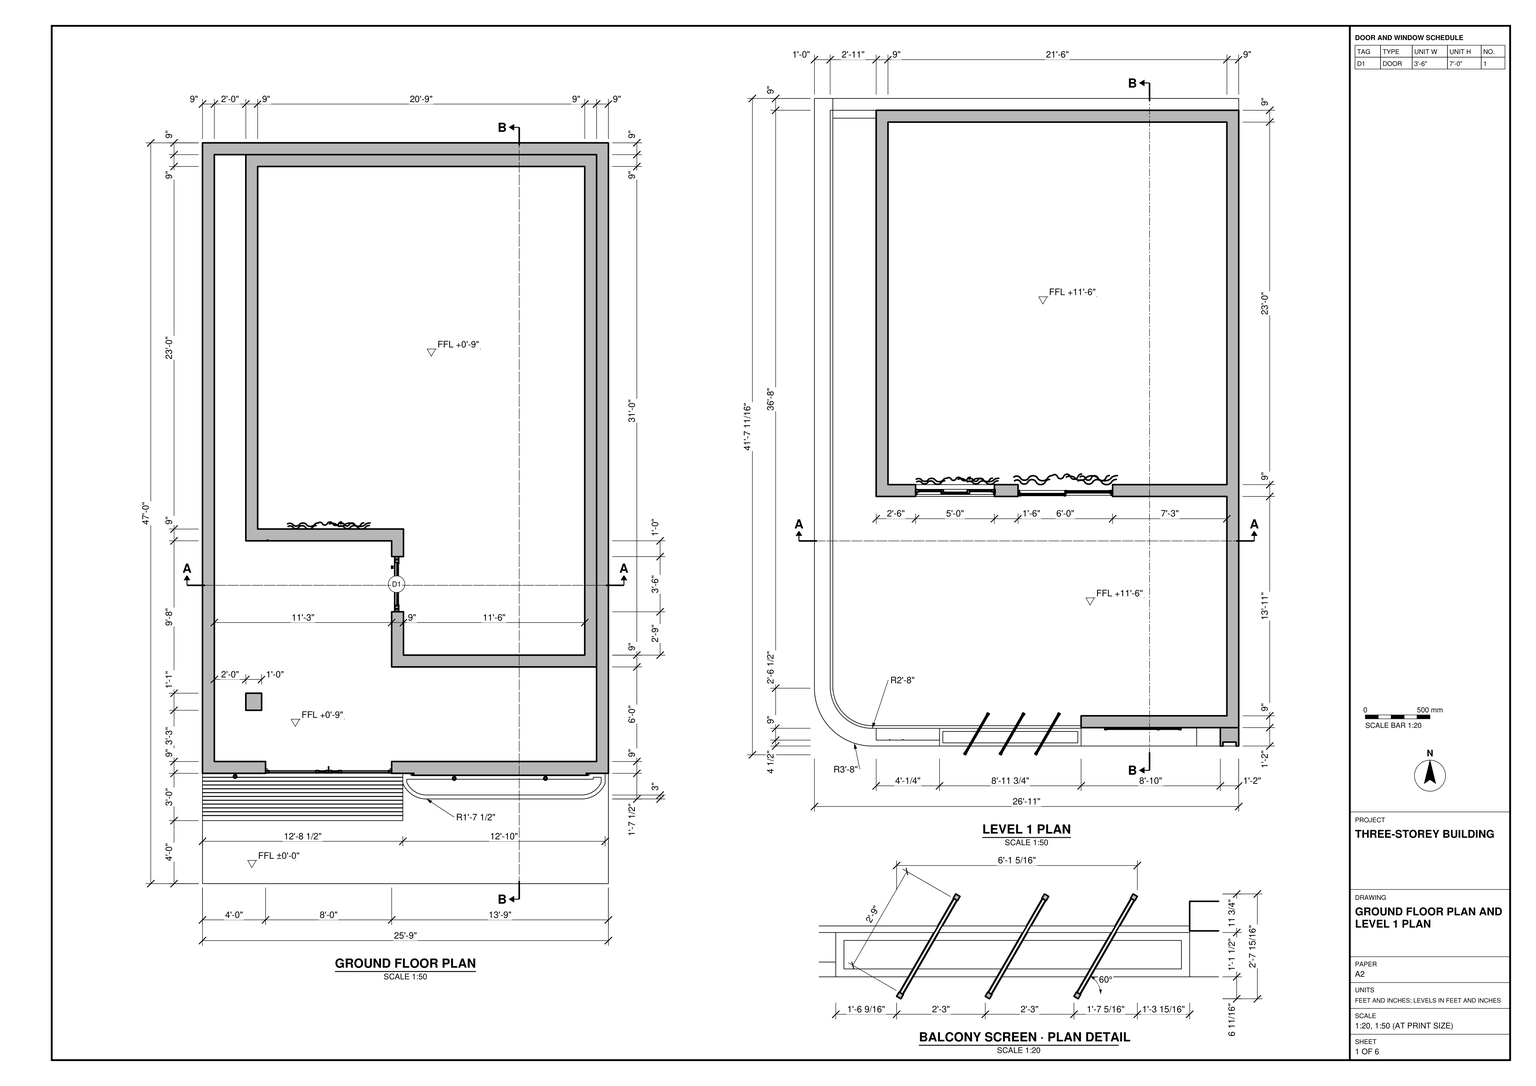
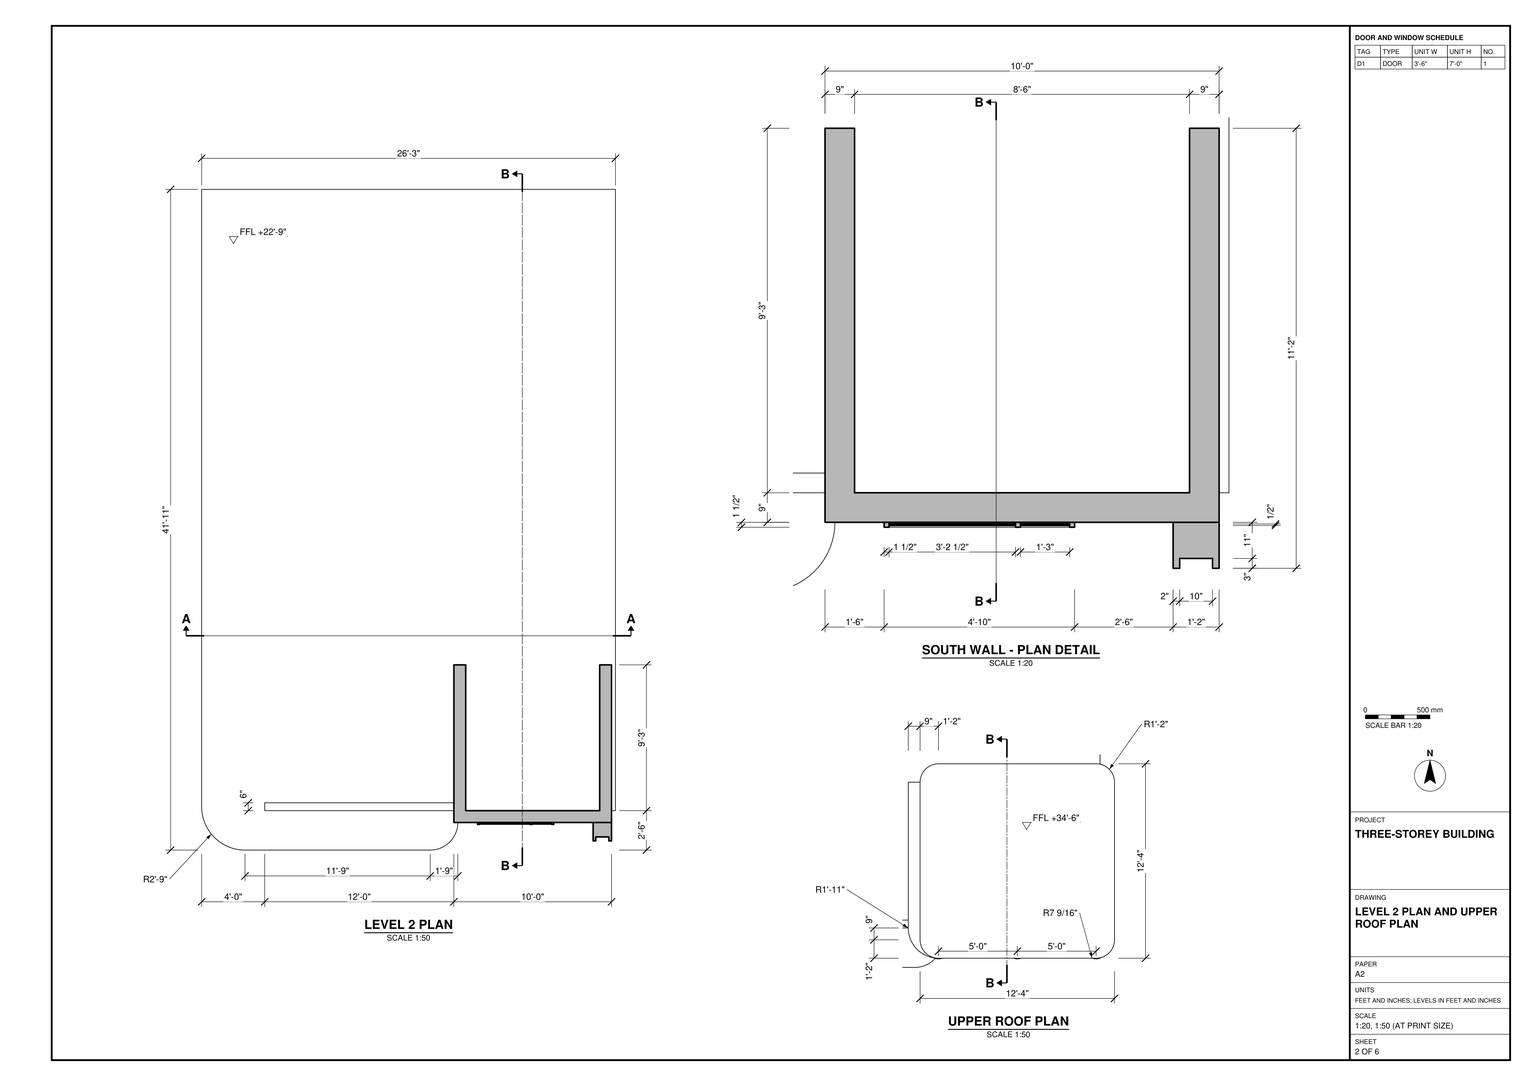
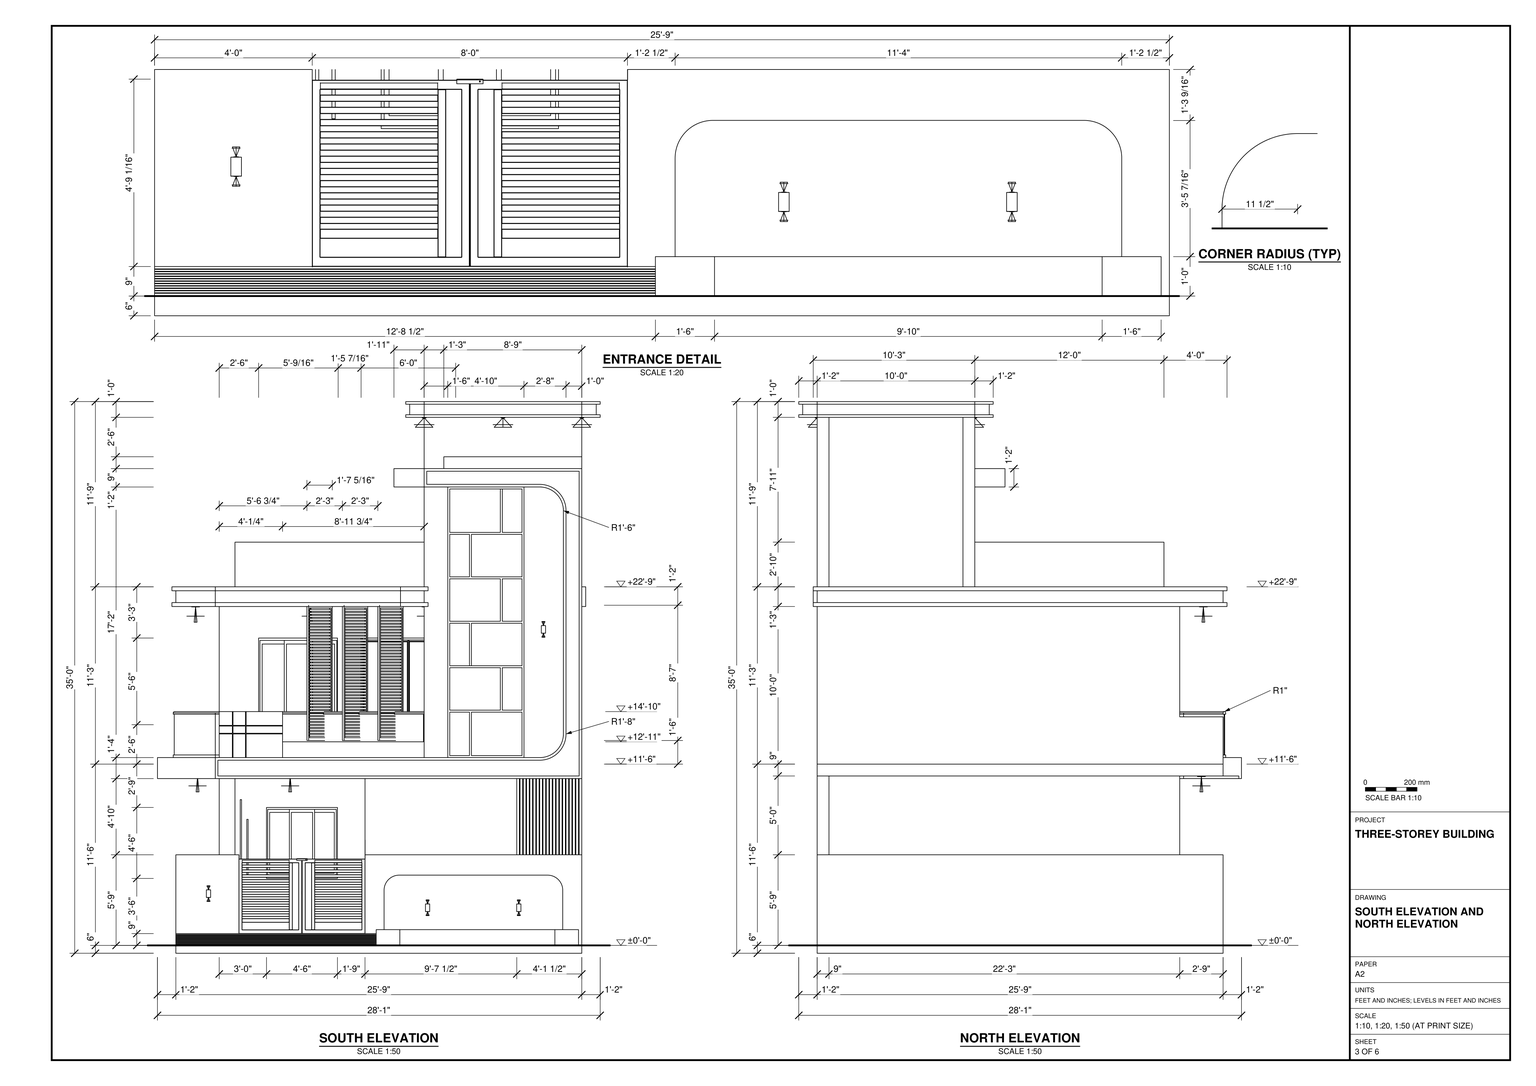
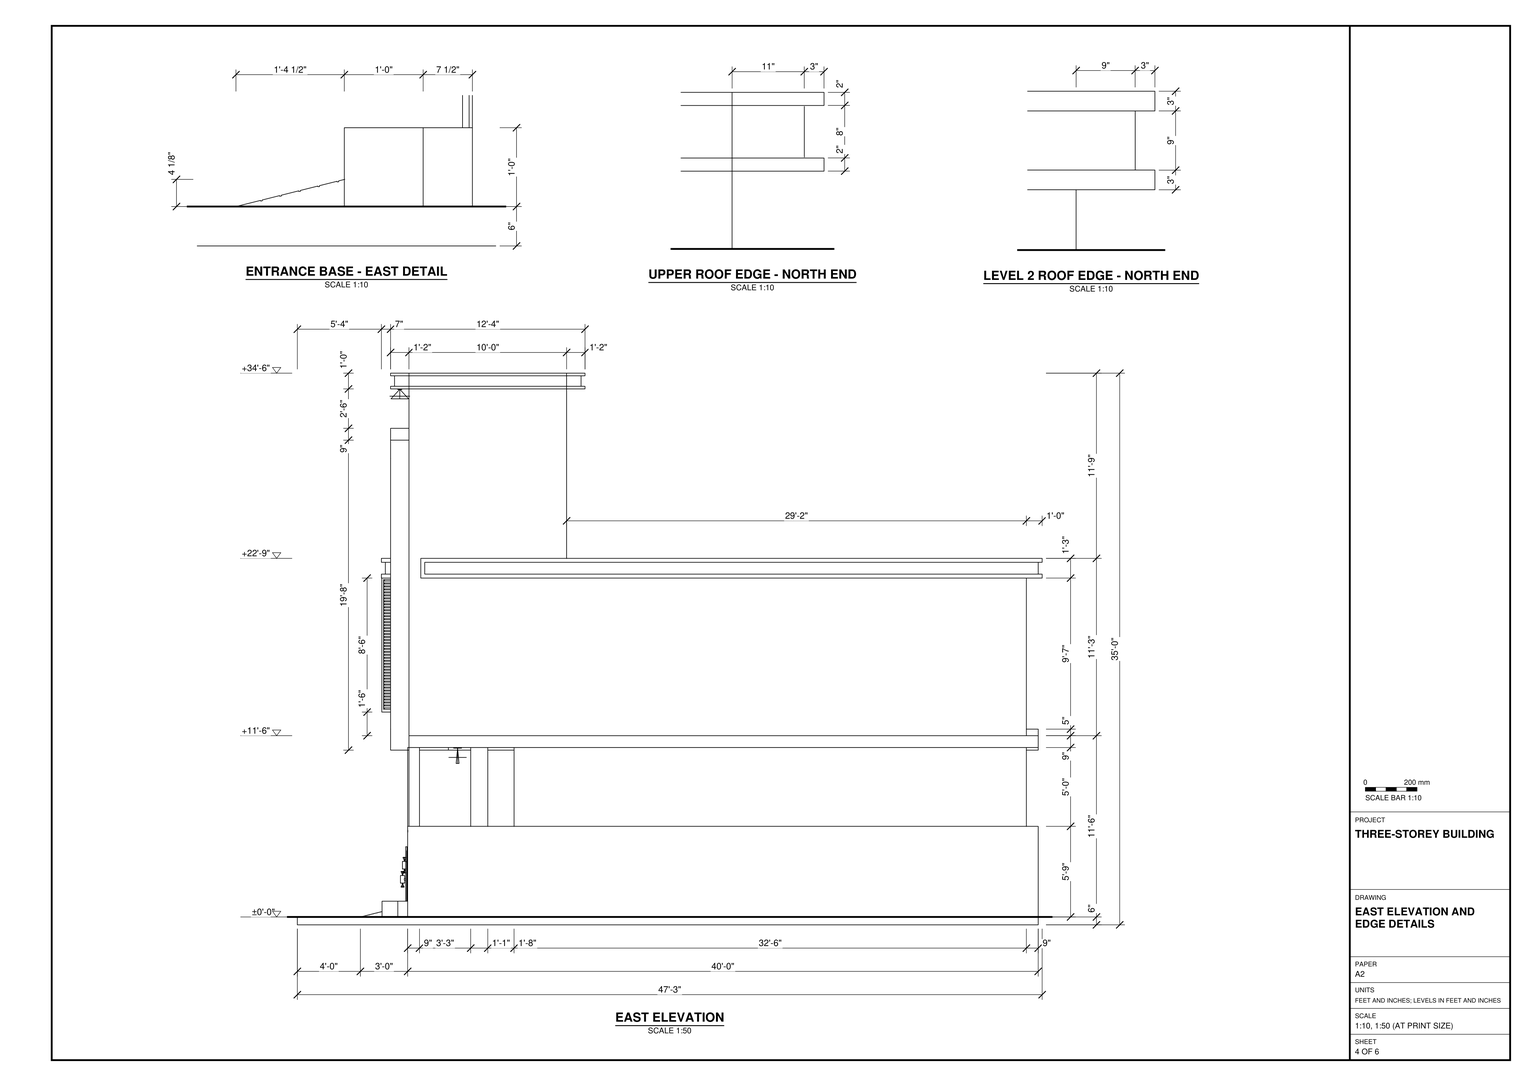
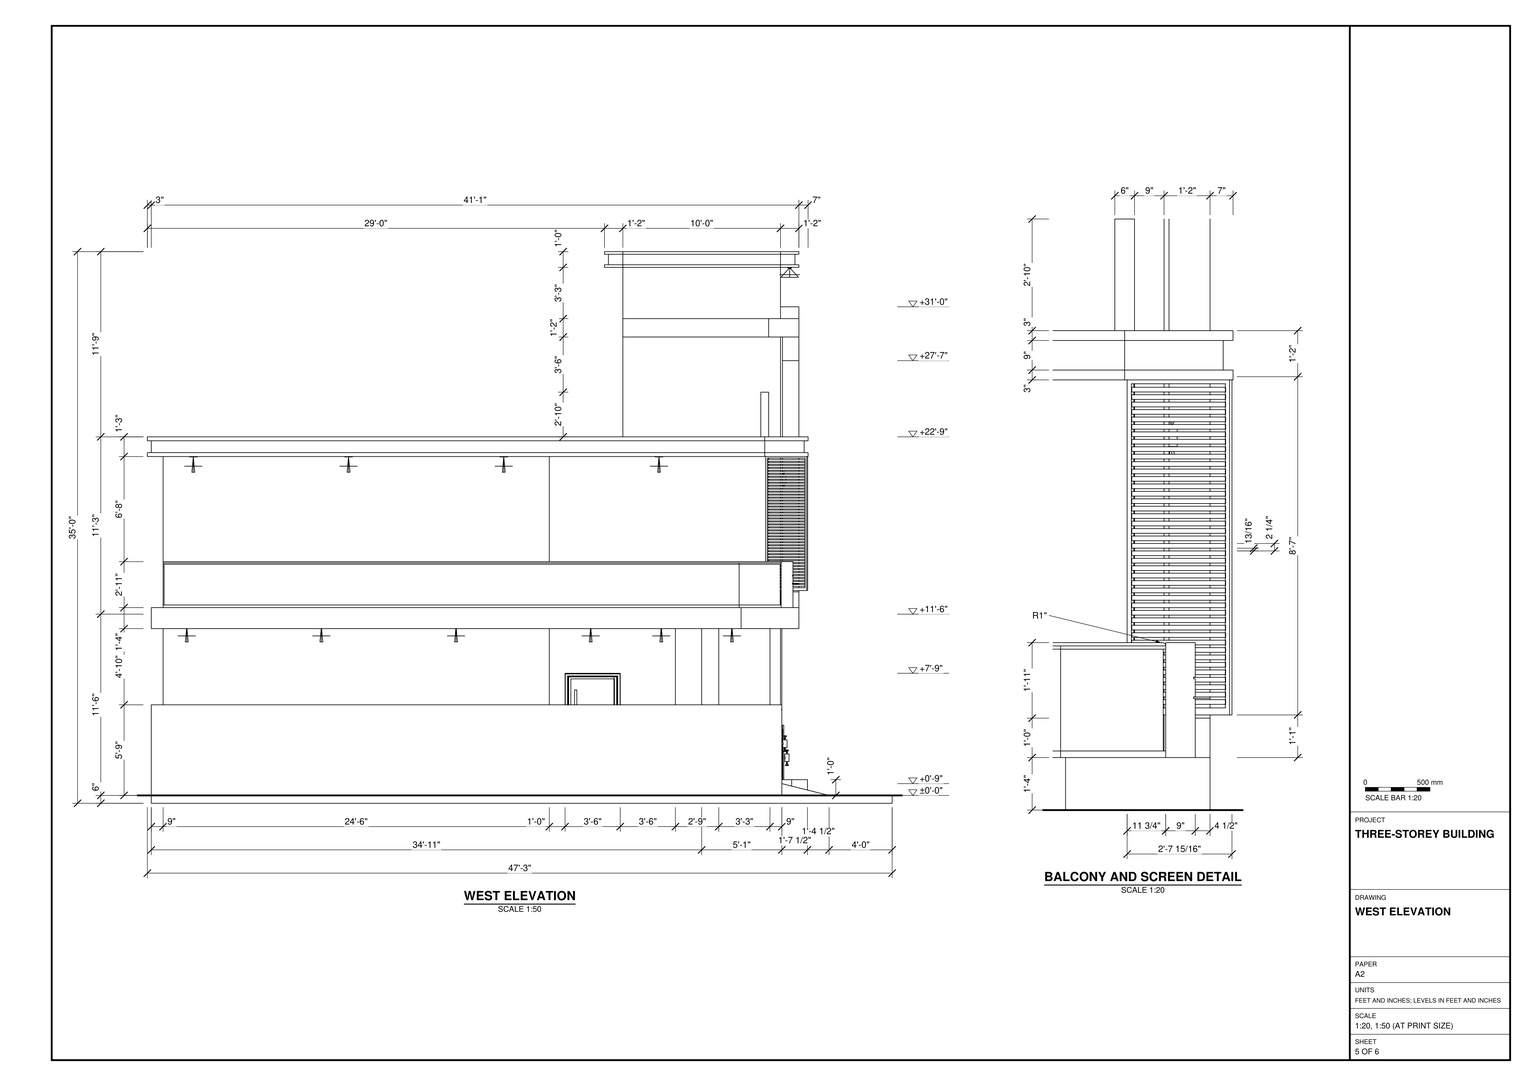
Build the three-storey building in SketchUp from task_files/diagram_01.pdf. Work in feet and inches. The overall model, including its projections, is 28'-1" wide, 47'-3" deep and 35'-0" high. Use ±0'-0" as the ground datum, with Level 1 at +11'-6" and Level 2 at +22'-9". Distinguish the raised ground-floor surface from the ground datum.

Follow the plan of each floor rather than repeating one footprint. Model the walls at their drawn thicknesses, including the 9" walls and the stepped ground-floor wall with a door in its return. On the south front, form the entrance steps, double slatted gate and adjoining low wall with its rounded-corner panel. Set the Level 1 enclosure back from the balcony. Include the window and door openings behind the balcony, the rounded slab corner, the railing and the angled slatted screens. Use the south elevation to place the tall panelled bay to the right of the screens and to shape its curved frame. At Level 2, model the broad roof deck and the smaller U-shaped wall at the front right, with its own overhanging roof cap.

Keep walls, slabs and roofs in separate groups or components. Group each furniture or joinery piece shown separately and use components for repeated parts. Decor and loose items, including light fixtures, may be any suitable library components. Save one SketchUp model as output_files/three_storey_building_with_a_screened_front_balcony.skp.

# SketchUp Ruby script. Lengths in inches.
U = 1.inch
M = Sketchup.active_model
def pt(a) = Geom::Point3d.new(a.map { |v| v * U })
def face(e, loops, mat)
  f = e.add_face(loops[0].map { |a| pt(a) })
  loops[1..].each { |l| e.add_face(l.map { |a| pt(a) }).erase! }
  f.material = f.back_material = mat if mat
  f
end
# faces: each face lists its corners as indices into pts; further lists are holes
def faces(e, pts, list, mat = nil) = list.each { |f| face(e, (f[0].is_a?(Array) ? f : [f]).map { |l| l.map { |i| pts[i] } }, mat) }
# xy, xz, yz: faces in a plane at the given z, y or x. An outline is a flat list of corners, or four numbers for a rectangle; further outlines are holes
def ring(l) = l.size == 4 ? [[l[0], l[1]], [l[2], l[1]], [l[2], l[3]], [l[0], l[3]]] : l.each_slice(2).to_a
def flat(e, list, mat, &to3) = list.each { |f| face(e, (f[0].is_a?(Array) ? f : [f]).map { |l| ring(l).map { |u, v| to3.(u, v) } }, mat) }
def xy(e, z, list, mat = nil) = flat(e, list, mat) { |x, y| [x, y, z] }
def xz(e, y, list, mat = nil) = flat(e, list, mat) { |x, z| [x, y, z] }
def yz(e, x, list, mat = nil) = flat(e, list, mat) { |y, z| [x, y, z] }
def lines(e, pts, list) = list.each { |a, b| e.add_line(pt(pts[a]), pt(pts[b])) }
# prism: a flat outline (further loops are holes) pulled along v
def prism(e, loops, v, mat = nil)
  f = face(e, loops, mat); d = Geom::Vector3d.new(v.map { |x| x * U })
  f.pushpull(f.normal.samedirection?(d) ? d.length : -d.length)
end
def box(e, o, s, mat = nil) = prism(e, [[o, [o[0] + s[0], o[1], o[2]], [o[0] + s[0], o[1] + s[1], o[2]], [o[0], o[1] + s[1], o[2]]]], [0, 0, s[2]], mat)
def at(x, y, z, deg = 0) = Geom::Transformation.translation(pt([x, y, z])) * Geom::Transformation.rotation(ORIGIN, Z_AXIS, deg.degrees)
def axes(o, x, y, z) = Geom::Transformation.new([*x, 0, *y, 0, *z, 0, *pt(o).to_a, 1])
def part(name) = M.definitions.add(name)
# library, detail: a bought-in or finely detailed component or shape, given as its bounding box
def library(name, o, s) = part(name).tap { |d| box(d.entities, o, s) }
def detail(e, o, s) = box(e.add_group.entities, o, s)
def put(e, d, t, mat = nil) = e.add_instance(d, t).tap { |i| i.material = mat if mat }
def group(e, t, mat = nil) = e.add_group.tap { |g| g.transformation = t; g.material = mat if mat }.entities
root = M.entities
M.materials.add("1496 AP 8293 CARBON COPY").color = [58, 58, 58]
M.materials.add("1755 AP K184 Brass Olive-N").color = [221, 212, 201]
M.materials.add("Antracyt").color = [44, 47, 50]
M.materials.add("Carpet_Frieze_Low").color = [170, 156, 146]
M.materials.add("Carpet_Loop_Low").color = [201, 172, 127]
M.materials.add("Wall Light").color = [248, 221, 148]
M.materials.add("[0135_DarkGray]").color = [81, 81, 81]
M.materials.add("[Basic Tile]").color = [188, 188, 188]
M.materials.add("[Carrera Marble]").color = [233, 230, 225]
M.materials.add("[Terrazzo Tile Light]").color = [178, 178, 178]
M.materials.add("[Translucent Glass Blue]").color = [169, 185, 212]
M.materials.add("[Translucent Glass Gray]").color = [128, 128, 128]
M.materials.add("[Wood Cherry Original]").color = [91, 49, 20]
M.materials.add("[Wood Cherry Original]1").color = [25, 25, 25]
c1 = library("2",[-4.69,-4.69,-13.16],[13.38,13.38,13.16])
c2 = library("WALL LIGHT 69",[4.19,4.05,-8.78],[4.61,5.7,17.13])
c3 = library("Group\#2",[0,-19.5,0],[309,499.5,129])
c4 = part("หน้าต่าง3บาน")
xy(c4.entities,42.78,[[77.6875,12.74,148.55,16.68]],"Antracyt")
xy(c4.entities,43.96,[[78.87,12.74,147.37,12.74,147.37,14.71,125.72,14.71,125.72,13.13,100.52,13.13,100.52,14.71,78.87,14.71],[100.52,13.13,102.88,14.71],[123.36,13.13,125.72,14.71],[102.49,14.71,123.75,14.71,123.75,16.28,147.37,16.28,147.37,16.68,78.87,16.68,78.87,16.28,102.49,16.28]],"Antracyt")
xy(c4.entities,45.93,[[102.49,13.13,123.75,13.92],[102.49,13.92,123.75,14.71],[80.84,14.71,100.52,15.49],[125.72,14.71,145.4,15.49],[80.84,15.49,100.52,16.28],
  [125.72,15.49,145.4,16.28]],"Antracyt")
xy(c4.entities,83.09,[[102.49,13.13,123.75,13.92],[102.49,13.92,123.75,14.71],[80.84,14.71,100.52,15.49],[125.72,14.71,145.4,15.49],[80.84,15.49,100.52,16.28],
  [125.72,15.49,145.4,16.28]],"Antracyt")
xy(c4.entities,84.91,[[78.87,12.74,78.87,14.71,100.52,14.71,100.52,13.13,125.72,13.13,125.72,14.71,147.37,14.71,147.37,12.74],[100.52,13.13,125.72,14.71],[102.49,14.71,102.49,16.28,78.87,16.28,78.87,16.68,147.37,16.68,147.37,16.28,123.75,16.28,123.75,14.71],[78.87,14.71,102.49,16.28]],"Antracyt")
xy(c4.entities,86.09,[[77.6875,12.74,148.55,16.68]],"Antracyt")
xz(c4.entities,12.74,[[[77.6875,42.78,148.55,86.09],[78.87,43.96,147.37,84.91]]],"Antracyt")
xz(c4.entities,13.13,[[[100.52,43.96,125.72,84.91],[102.49,45.93,123.75,83.09]]],"Antracyt")
xz(c4.entities,13.92,[[102.49,45.93,123.75,83.09]],"Antracyt")
xz(c4.entities,14.71,[[78.87,43.96,100.52,43.96,100.52,45.93,80.84,45.93,80.84,83.09,100.52,83.09,100.52,84.91,78.87,84.91],[100.52,43.96,102.49,84.91],[102.49,43.96,123.75,45.93],[125.72,43.96,147.37,43.96,147.37,84.91,125.72,84.91,125.72,83.09,145.4,83.09,145.4,45.93,125.72,45.93],[102.49,83.09,123.75,84.91]],"Antracyt")
xz(c4.entities,15.49,[[80.84,45.93,100.52,83.09],[125.72,45.93,145.4,83.09],[80.44,82.9375,80.84,83.73]],"Antracyt")
xz(c4.entities,16.28,[[[78.87,43.96,102.49,84.91],[80.84,45.93,100.52,83.09]],[[123.75,43.96,147.37,84.91],[125.72,45.93,145.4,83.09]]],"Antracyt")
xz(c4.entities,16.68,[[[77.6875,42.78,148.55,86.09],[78.87,43.96,147.37,84.91]]],"Antracyt")
yz(c4.entities,77.6875,[[12.74,42.78,16.68,86.09]],"Antracyt")
yz(c4.entities,78.87,[[12.74,43.96,14.71,84.91],[16.28,43.96,16.68,84.91]],"Antracyt")
yz(c4.entities,80.84,[[14.71,45.93,15.49,83.09],[15.49,45.93,16.28,83.09]],"Antracyt")
yz(c4.entities,100.52,[[13.13,43.96,14.71,84.91],[14.71,45.93,15.49,83.09],[15.49,45.93,16.28,83.09]],"Antracyt")
yz(c4.entities,102.49,[[14.71,43.96,16.28,84.91],[13.13,45.93,13.92,83.09],[13.92,45.93,14.71,83.09]],"Antracyt")
yz(c4.entities,123.75,[[14.71,43.96,16.28,84.91],[13.13,45.93,13.92,83.09],[13.92,45.93,14.71,83.09]],"Antracyt")
yz(c4.entities,125.72,[[13.13,43.96,14.71,84.91],[14.71,45.93,15.49,83.09],[15.49,45.93,16.28,83.09]],"Antracyt")
yz(c4.entities,145.4,[[14.71,45.93,15.49,83.09],[15.49,45.93,16.28,83.09]],"Antracyt")
yz(c4.entities,147.37,[[12.74,43.96,14.71,84.91],[16.28,43.96,16.68,84.91]],"Antracyt")
yz(c4.entities,148.55,[[12.74,42.78,16.68,86.09]],"Antracyt")
# 1 loose lines left out
c5 = library("Aluprof_MB-86_Drzwi_panelowe_003_S-0452",[0,0,0],[44.84,5.36,87])
c6 = part("Corrugated panel")
# 43 loose lines left out
p = [[17.625,0.0625,78.74],[17.625,0.0625,0],[18.27,0,0],[18.27,0,78.74],[18.92,0.0625,0],[18.92,0.0625,78.74],
  [17,0.25,78.74],[17,0.25,0],[19.55,0.25,0],[19.55,0.25,78.74],[16.43,0.56,78.74],[16.43,0.56,0],
  [20.12,0.56,0],[20.12,0.56,78.74],[6.31,0.6,78.74],[6.31,0.6,0],[6.8125,0.45,0],[6.8125,0.45,78.74],
  [7.33,0.4,0],[7.33,0.4,78.74],[7.86,0.45,0],[7.86,0.45,78.74],[8.36,0.6,0],[8.36,0.6,78.74],
  [5.85,0.85,78.74],[5.85,0.85,0],[8.82,0.85,0],[8.82,0.85,78.74],[15.92,0.97,78.74],[15.92,0.97,0],
  [20.625,0.97,0],[20.625,0.97,78.74],[5.44,1.18,78.74],[5.44,1.18,0],[9.23,1.18,0],[9.23,1.18,78.74],
  [15.51,1.48,78.74],[15.51,1.48,0],[21.04,1.48,0],[21.04,1.48,78.74],[5.11,1.59,78.74],[5.11,1.59,0],
  [9.5625,1.59,0],[9.5625,1.59,78.74],[14.93,2.55,78.74],[14.93,2.55,0],[15.2,2.04,0],[15.2,2.04,78.74],
  [21.34,2.04,0],[21.64,2.59,0],[21.64,2.59,78.74],[21.34,2.04,78.74],[4.63,2.47,78.74],[4.63,2.47,0],
  [4.86,2.04,0],[4.86,2.04,78.74],[9.81,2.04,0],[10.08,2.55,0],[10.08,2.55,78.74],[9.81,2.04,78.74],
  [4.32,2.85,78.74],[4.32,2.85,0],[10.44,2.99,0],[10.44,2.99,78.74],[14.57,2.99,78.74],[14.57,2.99,0],
  [22.03,3.0625,0],[22.03,3.0625,78.74],[0.85,2.85,78.74],[0.85,2.85,0],[1.22,3.15,0],[1.22,3.15,78.74],
  [3.95,3.15,78.74],[3.95,3.15,0],[10.89,3.35,0],[10.89,3.35,78.74],[14.125,3.35,78.74],[14.125,3.35,0],
  [22.5,3.45,0],[22.5,3.45,78.74],[1.65,3.375,0],[1.65,3.375,78.74],[3.53,3.375,78.74],[3.53,3.375,0],
  [2.11,3.52,0],[2.11,3.52,78.74],[3.07,3.52,78.74],[3.07,3.52,0],[11.39,3.625,0],[11.39,3.625,78.74],
  [13.62,3.625,78.74],[13.62,3.625,0],[2.59,3.5625,0],[2.59,3.5625,78.74],[23.04,3.74,0],[23.04,3.74,78.74],
  [11.9375,3.79,0],[11.9375,3.79,78.74],[13.07,3.79,78.74],[13.07,3.79,0],[23.63,3.92,0],[23.63,3.92,78.74],
  [12.51,3.85,0],[12.51,3.85,78.74],[24.25,3.98,0],[24.25,3.98,78.74]]
faces(c6.entities,p,[[0,1,2,3],[3,2,4,5],[6,7,1,0],[5,4,8,9],[10,11,7,6],[9,8,12,13],[14,15,16,17],[17,16,18,19],
  [19,18,20,21],[21,20,22,23],[24,25,15,14],[23,22,26,27],[28,29,11,10],[13,12,30,31],[32,33,25,24],[27,26,34,35],
  [36,37,29,28],[31,30,38,39],[40,41,33,32],[35,34,42,43],[44,45,46,37,36,47],[39,38,48,49,50,51],[52,53,54,41,40,55],[43,42,56,57,58,59],
  [60,61,53,52],[58,57,62,63],[64,65,45,44],[50,49,66,67],[68,69,70,71],[72,73,61,60],[63,62,74,75],[76,77,65,64],
  [67,66,78,79],[71,70,80,81],[82,83,73,72],[81,80,84,85],[86,87,83,82],[75,74,88,89],[90,91,77,76],[85,84,92,93],
  [93,92,87,86],[79,78,94,95],[89,88,96,97],[98,99,91,90],[95,94,100,101],[97,96,102,103],[103,102,99,98],[101,100,104,105]])
c7 = part("Tubular post section")
yz(c7.entities,0,[[1.55,0.61,1.31,0.64,1.08,0.73,0.88,0.88,0.73,1.08,0.64,1.31,0.61,1.55,0.64,1.79,0.73,2.02,0.88,2.22,1.08,2.37,1.31,2.46,1.55,2.49,1.79,2.46,2.02,2.37,2.22,2.22,2.37,2.02,2.46,1.79,2.49,1.55,2.46,1.31,2.37,1.08,2.22,0.88,2.02,0.73,1.79,0.64]])
yz(c7.entities,2.36,[[[1.55,0,1.15,0.05,0.78,0.21,0.45,0.45,0.21,0.78,0.05,1.15,0,1.55,0.05,1.95,0.21,2.33,0.45,2.65,0.78,2.89,1.15,3.05,1.55,3.1,1.95,3.05,2.33,2.89,2.65,2.65,2.89,2.33,3.05,1.95,3.1,1.55,3.05,1.15,2.89,0.78,2.65,0.45,2.33,0.21,1.95,0.05],[1.55,0.61,1.79,0.64,2.02,0.73,2.22,0.88,2.37,1.08,2.46,1.31,2.49,1.55,2.46,1.79,2.37,2.02,2.22,2.22,2.02,2.37,1.79,2.46,1.55,2.49,1.31,2.46,1.08,2.37,0.88,2.22,0.73,2.02,0.64,1.79,0.61,1.55,0.64,1.31,0.73,1.08,0.88,0.88,1.08,0.73,1.31,0.64]]])
yz(c7.entities,3.15,[[[1.55,0,1.95,0.05,2.33,0.21,2.65,0.45,2.89,0.78,3.05,1.15,3.1,1.55,3.05,1.95,2.89,2.33,2.65,2.65,2.33,2.89,1.95,3.05,1.55,3.1,1.15,3.05,0.78,2.89,0.45,2.65,0.21,2.33,0.05,1.95,0,1.55,0.05,1.15,0.21,0.78,0.45,0.45,0.78,0.21,1.15,0.05],[1.55,0.61,1.31,0.64,1.08,0.73,0.88,0.88,0.73,1.08,0.64,1.31,0.61,1.55,0.64,1.79,0.73,2.02,0.88,2.22,1.08,2.37,1.31,2.46,1.55,2.49,1.79,2.46,2.02,2.37,2.22,2.22,2.37,2.02,2.46,1.79,2.49,1.55,2.46,1.31,2.37,1.08,2.22,0.88,2.02,0.73,1.79,0.64]]])
yz(c7.entities,37.22,[[1.55,0.61,1.79,0.64,2.02,0.73,2.22,0.88,2.37,1.08,2.46,1.31,2.49,1.55,2.46,1.79,2.37,2.02,2.22,2.22,2.02,2.37,1.79,2.46,1.55,2.49,1.31,2.46,1.08,2.37,0.88,2.22,0.73,2.02,0.64,1.79,0.61,1.55,0.64,1.31,0.73,1.08,0.88,0.88,1.08,0.73,1.31,0.64]])
p = [[2.36,1.15,0.05],[2.36,1.55,0],[3.15,1.55,0],[3.15,1.15,0.05],[2.36,1.95,0.05],[3.15,1.95,0.05],
  [2.36,0.78,0.21],[3.15,0.78,0.21],[2.36,2.33,0.21],[3.15,2.33,0.21],[2.36,0.45,0.45],[3.15,0.45,0.45],
  [2.36,2.65,0.45],[3.15,2.65,0.45],[2.36,0.21,0.78],[3.15,0.21,0.78],[2.36,2.89,0.78],[3.15,2.89,0.78],
  [2.36,1.31,0.64],[2.36,1.08,0.73],[0,1.08,0.73],[0,1.31,0.64],[3.15,1.31,0.64],[3.15,1.08,0.73],
  [37.22,1.31,0.64],[37.22,1.08,0.73],[2.36,1.55,0.61],[0,1.55,0.61],[3.15,1.55,0.61],[37.22,1.55,0.61],
  [2.36,1.79,0.64],[0,1.79,0.64],[3.15,1.79,0.64],[37.22,1.79,0.64],[2.36,2.02,0.73],[0,2.02,0.73],
  [3.15,2.02,0.73],[37.22,2.02,0.73],[2.36,0.88,0.88],[0,0.88,0.88],[3.15,0.88,0.88],[37.22,0.88,0.88],
  [2.36,2.22,0.88],[0,2.22,0.88],[3.15,2.22,0.88],[37.22,2.22,0.88],[2.36,0.05,1.15],[3.15,0.05,1.15],
  [2.36,3.05,1.15],[3.15,3.05,1.15],[2.36,0.73,1.08],[0,0.73,1.08],[3.15,0.73,1.08],[37.22,0.73,1.08],
  [2.36,2.37,1.08],[0,2.37,1.08],[3.15,2.37,1.08],[37.22,2.37,1.08],[2.36,0,1.55],[3.15,0,1.55],
  [2.36,0.64,1.31],[0,0.64,1.31],[3.15,0.64,1.31],[37.22,0.64,1.31],[2.36,2.46,1.31],[0,2.46,1.31],
  [3.15,2.46,1.31],[37.22,2.46,1.31],[2.36,3.1,1.55],[3.15,3.1,1.55],[2.36,0.61,1.55],[0,0.61,1.55],
  [3.15,0.61,1.55],[37.22,0.61,1.55],[2.36,2.49,1.55],[0,2.49,1.55],[3.15,2.49,1.55],[37.22,2.49,1.55],
  [2.36,0.05,1.95],[3.15,0.05,1.95],[2.36,0.64,1.79],[0,0.64,1.79],[3.15,0.64,1.79],[37.22,0.64,1.79],
  [2.36,2.46,1.79],[0,2.46,1.79],[3.15,2.46,1.79],[37.22,2.46,1.79],[2.36,3.05,1.95],[3.15,3.05,1.95],
  [2.36,0.73,2.02],[0,0.73,2.02],[3.15,0.73,2.02],[37.22,0.73,2.02],[2.36,2.37,2.02],[0,2.37,2.02],
  [3.15,2.37,2.02],[37.22,2.37,2.02],[2.36,0.21,2.33],[3.15,0.21,2.33],[2.36,0.88,2.22],[0,0.88,2.22],
  [3.15,0.88,2.22],[37.22,0.88,2.22],[2.36,2.22,2.22],[0,2.22,2.22],[3.15,2.22,2.22],[37.22,2.22,2.22],
  [2.36,2.89,2.33],[3.15,2.89,2.33],[2.36,1.08,2.37],[0,1.08,2.37],[3.15,1.08,2.37],[37.22,1.08,2.37],
  [2.36,2.02,2.37],[0,2.02,2.37],[3.15,2.02,2.37],[37.22,2.02,2.37],[2.36,0.45,2.65],[3.15,0.45,2.65],
  [2.36,2.65,2.65],[3.15,2.65,2.65],[2.36,1.31,2.46],[0,1.31,2.46],[3.15,1.31,2.46],[37.22,1.31,2.46],
  [2.36,1.79,2.46],[0,1.79,2.46],[3.15,1.79,2.46],[37.22,1.79,2.46],[2.36,1.55,2.49],[0,1.55,2.49],
  [3.15,1.55,2.49],[37.22,1.55,2.49],[2.36,0.78,2.89],[3.15,0.78,2.89],[2.36,2.33,2.89],[3.15,2.33,2.89],
  [2.36,1.15,3.05],[3.15,1.15,3.05],[2.36,1.95,3.05],[3.15,1.95,3.05],[2.36,1.55,3.1],[3.15,1.55,3.1]]
faces(c7.entities,p,[[0,1,2,3],[1,4,5,2],[6,0,3,7],[4,8,9,5],[10,6,7,11],[8,12,13,9],[14,10,11,15],[12,16,17,13],
  [18,19,20,21],[19,18,22,23],[24,25,23,22],[26,18,21,27],[18,26,28,22],[29,24,22,28],[30,26,27,31],[26,30,32,28],
  [33,29,28,32],[34,30,31,35],[30,34,36,32],[37,33,32,36],[19,38,39,20],[38,19,23,40],[25,41,40,23],[42,34,35,43],
  [34,42,44,36],[45,37,36,44],[46,14,15,47],[16,48,49,17],[38,50,51,39],[50,38,40,52],[41,53,52,40],[54,42,43,55],
  [42,54,56,44],[57,45,44,56],[58,46,47,59],[50,60,61,51],[60,50,52,62],[53,63,62,52],[64,54,55,65],[54,64,66,56],
  [67,57,56,66],[48,68,69,49],[60,70,71,61],[70,60,62,72],[63,73,72,62],[74,64,65,75],[64,74,76,66],[77,67,66,76],
  [78,58,59,79],[70,80,81,71],[80,70,72,82],[73,83,82,72],[84,74,75,85],[74,84,86,76],[87,77,76,86],[68,88,89,69],
  [80,90,91,81],[90,80,82,92],[83,93,92,82],[94,84,85,95],[84,94,96,86],[97,87,86,96],[98,78,79,99],[90,100,101,91],
  [100,90,92,102],[93,103,102,92],[104,94,95,105],[94,104,106,96],[107,97,96,106],[88,108,109,89],[100,110,111,101],[110,100,102,112],
  [103,113,112,102],[114,104,105,115],[104,114,116,106],[117,107,106,116],[118,98,99,119],[108,120,121,109],[110,122,123,111],[122,110,112,124],
  [113,125,124,112],[126,114,115,127],[114,126,128,116],[129,117,116,128],[122,130,131,123],[130,122,124,132],[125,133,132,124],[130,126,127,131],
  [126,130,132,128],[133,129,128,132],[134,118,119,135],[120,136,137,121],[138,134,135,139],[136,140,141,137],[142,138,139,143],[140,142,143,141]])
c8 = part("Tubular post")
put(c8.entities,c7,axes([3.125,-0.76,-2.47],[0,0,1.25313],[0,1.25313,0],[-1.25313,0,0]))
put(c8.entities,c7,axes([3.125,3.125,81],[0,0,-1.25313],[0,-1.25313,0],[-1.25313,0,0]))
c9 = part("Untitled")
p = [[59.99,12.8,78.74],[59.99,12.8,0],[60.15,12.52,0],[60.15,12.52,78.74],[66.72,13.7,0],[66.72,13.7,78.74],
  [73.91,13.97,78.74],[73.91,13.97,0],[49.31,14.13,0],[49.31,14.13,78.74]]
lines(c9.entities,p,[[0,1],[2,3],[4,5],[6,7],[8,9]])
put(c9.entities,c6,axes([64.94,10.15,0],[0.73,0,0],[0,1,0],[0,0,1]),"Carpet_Loop_Low")
put(c9.entities,c6,axes([48.6875,11.28,0],[0.73,0,0],[0,1,0],[0,0,1]),"Carpet_Loop_Low")
put(c9.entities,c6,axes([25.83,10.15,0],[0.96815,0,0],[0,1,0],[0,0,1]),"Carpet_Loop_Low")
put(c9.entities,c6,axes([56.28,10.09,0],[1.28298,0,0],[0,1,0],[0,0,1]),"Carpet_Loop_Low")
put(c9.entities,c8,axes([25.47,12.88,78.42],[0,0,-0.798],[0,0.798,0],[0.798,0,0]))
g1 = group(c9.entities,at(27.05,7.18,0))
put(g1,c6,axes([-0.75,0,0],[0.87994,0,0],[0,1,0],[0,0,1]),"Carpet_Frieze_Low")
put(g1,c6,axes([36.48,0,0],[0.95864,0,0],[0,1,0],[0,0,1]),"Carpet_Frieze_Low")
c10 = part("PENTEK_RP Fineline 50S_Sliding_DoorCase_E1")
box(c10.entities,[0,0,0],[1.51,3.66,99.27],"[0135_DarkGray]")
c11 = part("PENTEK_RP Fineline 50S_SlidingDooe_Case_E2")
box(c11.entities,[0,0,0],[96.25,3.66,1.51],"[0135_DarkGray]")
c12 = part("pentek_RP Fineline 50S_SlidingDoor_Case")
put(c12.entities,c10,at(97.76,0,0))
put(c12.entities,c11,at(1.51,0,0))
put(c12.entities,c10,at(0,0,0))
put(c12.entities,c11,at(1.51,0,97.76))
c13 = part("PENTEK_RP Fineline 50S_SlidingDoor_GlazingBead_2")
box(c13.entities,[0,0,0],[0.56,0.59,94.39],"[0135_DarkGray]")
c14 = part("PENTEK_RP Fineline 50S_SlidingDoor_Glass")
box(c14.entities,[0,0,0],[46.58,0.16,94.39],"[Translucent Glass Gray]")
c15 = part("PENTEK_RP Fineline 50S_SlidingDoor_GlazingBead")
box(c15.entities,[0,0,0],[45.47,0.59,0.56],"[0135_DarkGray]")
c16 = part("PENTEK_RP Fineline 50S_SlidingDoor_Leaf_E1")
xy(c16.entities,0,[[0,0,0.93,1.97],[0.93,1.57,1.49,1.97]],"[0135_DarkGray]")
xy(c16.entities,96.25,[[0,0,0.93,0,0.93,1.57,1.49,1.57,1.49,1.97,0,1.97]],"[0135_DarkGray]")
xz(c16.entities,0,[[0,0,0.93,96.25]],"[0135_DarkGray]")
xz(c16.entities,1.57,[[0.93,0,1.49,95.32],[0.93,95.32,1.49,96.25]],"[0135_DarkGray]")
xz(c16.entities,1.97,[[0,0,1.49,96.25]],"[0135_DarkGray]")
yz(c16.entities,0,[[0,0,1.97,96.25]],"[0135_DarkGray]")
yz(c16.entities,0.93,[[0,0,1.57,0.93],[0,0.93,1.57,95.32],[0,95.32,1.57,96.25]],"[0135_DarkGray]")
yz(c16.entities,1.49,[[1.57,0,1.97,95.32],[1.57,95.32,1.97,96.25]],"[0135_DarkGray]")
c17 = part("PENTEK_RP Fineline 50S_SlidingDoor_Leaf_E2")
xy(c17.entities,0,[[0,0,0,1.57,0.56,1.57,0.56,1.97,46.02,1.97,46.02,1.57,46.58,1.57,46.58,0]],"[0135_DarkGray]")
xy(c17.entities,0.93,[[0,0,46.58,1.57]],"[0135_DarkGray]")
xy(c17.entities,1.49,[[0.56,1.57,46.02,1.97]],"[0135_DarkGray]")
xz(c17.entities,0,[[0,0,46.58,0.93]],"[0135_DarkGray]")
xz(c17.entities,1.57,[[0,0,0.56,0.93],[46.02,0,46.58,0.93],[0.56,0.93,46.02,1.49]],"[0135_DarkGray]")
xz(c17.entities,1.97,[[0.56,0,46.02,1.49]],"[0135_DarkGray]")
yz(c17.entities,0,[[0,0,1.57,0.93]],"[0135_DarkGray]")
yz(c17.entities,0.56,[[1.57,0,1.97,0.93],[1.57,0.93,1.97,1.49]],"[0135_DarkGray]")
yz(c17.entities,46.02,[[1.57,0,1.97,0.93],[1.57,0.93,1.97,1.49]],"[0135_DarkGray]")
yz(c17.entities,46.58,[[0,0,1.57,0.93]],"[0135_DarkGray]")
c18 = part("PENTEK_RP Fineline S_SlidingDoor_Leaf1")
put(c18.entities,c13,at(0.93,0,0.93))
put(c18.entities,c13,at(46.96,0,0.93))
put(c18.entities,c14,at(1.49,1.42,0.93))
put(c18.entities,c15,at(1.49,0,0.93))
put(c18.entities,c14,at(1.49,0.59,0.93))
put(c18.entities,c16,at(0,0,0))
put(c18.entities,c16,axes([48.44,0,0],[-1,0,0],[0,1,0],[0,0,1]))
put(c18.entities,c17,axes([0.93,0,96.25],[1,0,0],[0,1,0],[0,0,-1]))
put(c18.entities,c17,at(0.93,0,0))
put(c18.entities,c15,at(1.49,0,94.77))
c19 = part("PENTEK_RP Fineline 50S_SlidingDoor_Leaf2")
put(c19.entities,c14,at(1.49,1.42,0.93))
put(c19.entities,c15,at(1.49,0,94.77))
put(c19.entities,c13,at(46.96,0,0.93))
put(c19.entities,c14,at(1.49,0.59,0.93))
put(c19.entities,c13,at(0.93,0,0.93))
put(c19.entities,c16,at(0,0,0))
put(c19.entities,c16,axes([48.44,0,0],[-1,0,0],[0,1,0],[0,0,1]))
put(c19.entities,c15,at(1.49,0,0.93))
put(c19.entities,c17,axes([0.93,0,96.25],[1,0,0],[0,1,0],[0,0,-1]))
put(c19.entities,c17,at(0.93,0,0))
c20 = part("PENTEK_RP+Fineline+50S_Sliding_Door (1)")
put(c20.entities,c12,at(0,-1.88,-0.09))
put(c20.entities,c18,at(1.51,-2.27,1.42))
put(c20.entities,c19,at(49.32,-0.3,1.42))
c21 = library("Group\#13",[-3,-21,-14.96],[315,503,26.96])
c22 = library("Group\#8",[-14,-20.68,-2],[323,499.68,245])
c23 = library("Group\#14",[-14,-14.57,-7.55],[148,148.57,19.55])
g2 = group(root,at(0,84,0))
box(g2,[33,48,9],[12,13,120],"1496 AP 8293 CARBON COPY")
put(g2,c1,at(14.5,143.5,130.01))
put(g2,c1,at(14.5,89.75,130.01))
put(g2,c1,at(14.5,36,130.01))
put(g2,c1,at(14.5,246,130.01))
put(g2,c1,at(14.5,348.5,130.01))
put(g2,c1,at(14.5,451,130.01))
put(g2,c1,at(85,143.5,130.01))
put(g2,c1,at(85,36,130.01))
put(g2,c1,at(85,89.75,130.01))
put(g2,c1,at(184,36,130.01))
put(g2,c1,at(283,36,130.01))
put(g2,c2,axes([187.07,-8.32,28.83],[0.7,0,0],[0,0.7,0],[0,0,0.7]))
put(g2,c2,axes([256.51,-8.32,28.83],[0.7,0,0],[0,0.7,0],[0,0,0.7]))
put(g2,c2,axes([20.29,-6.82,39.58],[0.7,0,0],[0,0.7,0],[0,0,0.7]))
put(g2,c2,axes([275.27,-5.82,240.75],[0.7,0,0],[0,0.7,0],[0,0,0.7]))
put(g2,c3,at(0,0,0))
g3 = group(g2,at(9,9,0))
xy(g3,0,[[39,-9,39,0,0,0,0,462,291,462,291,0,135,0,135,-9]])
xy(g3,9,[[39,-9,135,-9,135,0,291,0,291,462,0,462,0,0,39,0]],"[Terrazzo Tile Light]")
xz(g3,-9,[[39,0,135,9]])
xz(g3,0,[[0,0,39,9],[135,0,291,9]])
xz(g3,462,[[0,0,291,9]])
yz(g3,0,[[0,0,462,9]])
yz(g3,39,[[-9,0,0,9]])
yz(g3,135,[[-9,0,0,9]])
yz(g3,291,[[0,0,462,9]])
g4 = group(g2,at(9,81,9))
xy(g4,0,[[135,0,135,42,144,42,144,9,282,9,282,381,33,381,33,105,144,105,144,84,135,84,135,96,24,96,24,390,291,390,291,0]],"1755 AP K184 Brass Olive-N")
xy(g4,28,[[40,96,41,96.5]],"1755 AP K184 Brass Olive-N")
xy(g4,42,[[60,96,114,105]],"1755 AP K184 Brass Olive-N")
xy(g4,45,[[45,96,46,96.5]],"1755 AP K184 Brass Olive-N")
xy(g4,84,[[135,42,144,84]],"1755 AP K184 Brass Olive-N")
xy(g4,87,[[45,96,46,96.5]],"1755 AP K184 Brass Olive-N")
xy(g4,96,[[60,96,114,105]],"1755 AP K184 Brass Olive-N")
xy(g4,102,[[40,96,41,96.5]],"1755 AP K184 Brass Olive-N")
xy(g4,120,[[[135,0,291,0,291,390,24,390,24,96,135,96],[144,9,144,105,33,105,33,381,282,381,282,9]]],"1755 AP K184 Brass Olive-N")
xz(g4,0,[[135,0,291,120]],"1755 AP K184 Brass Olive-N")
xz(g4,9,[[144,0,282,120]],"1755 AP K184 Brass Olive-N")
xz(g4,42,[[135,0,144,84]],"1755 AP K184 Brass Olive-N")
xz(g4,84,[[135,0,144,84]],"1755 AP K184 Brass Olive-N")
xz(g4,96,[[[24,0,135,120],[60,42,114,96],[40,28,41,102],[45,45,46,87]]],"1755 AP K184 Brass Olive-N")
xz(g4,96.5,[[40,28,41,102],[45,45,46,87]],"1755 AP K184 Brass Olive-N")
xz(g4,105,[[[33,0,144,120],[60,42,114,96]]],"1755 AP K184 Brass Olive-N")
xz(g4,381,[[33,0,282,120]],"1755 AP K184 Brass Olive-N")
xz(g4,390,[[24,0,291,120]],"1755 AP K184 Brass Olive-N")
yz(g4,24,[[96,0,390,120]],"1755 AP K184 Brass Olive-N")
yz(g4,33,[[105,0,381,120]],"1755 AP K184 Brass Olive-N")
yz(g4,40,[[96,28,96.5,102]],"1755 AP K184 Brass Olive-N")
yz(g4,41,[[96,28,96.5,102]],"1755 AP K184 Brass Olive-N")
yz(g4,45,[[96,45,96.5,87]],"1755 AP K184 Brass Olive-N")
yz(g4,46,[[96,45,96.5,87]],"1755 AP K184 Brass Olive-N")
yz(g4,60,[[96,42,105,96]],"1755 AP K184 Brass Olive-N")
yz(g4,114,[[96,42,105,96]],"1755 AP K184 Brass Olive-N")
yz(g4,135,[[0,0,0,120,96,120,96,0,84,0,84,84,42,84,42,0]],"1755 AP K184 Brass Olive-N")
yz(g4,144,[[9,0,42,0,42,84,84,84,84,0,105,0,105,120,9,120]],"1755 AP K184 Brass Olive-N")
yz(g4,282,[[9,0,381,120]],"1755 AP K184 Brass Olive-N")
yz(g4,291,[[0,0,390,120]],"1755 AP K184 Brass Olive-N")
put(g4,c4,axes([0.8,84.51,-11.34],[0.762,0,0],[0,1,0],[0,0,1.24691]))
put(g4,c5,axes([135,84,0],[0,-0.93661,0],[1,0,0],[0,0,0.96551]))
put(g4,c9,axes([28.15,100.19,27.32],[1.03545,0,0],[0,0.67,0],[0,0,0.96547]))
g5 = group(g4,at(38,96.5,28),"Wall Light")
box(g5,[2,-0.5,0],[1,0.5,74])
box(g5,[7,-0.5,17],[1,0.5,42])
g6 = group(g2,at(33,177,138))
xy(g6,0,[[156,-176,156,-167,267,-167,267,0,180,0,180,9,267,9,267,285,9,285,9,9,108,9,108,0,0,0,0,288,-33,288,-33,294,276,294,276,-176]])
xy(g6,30,[[30,0,90,9]])
xy(g6,36,[[-33,288,0,294]])
xy(g6,96,[[30,0,90,9],[108,0,180,9]])
xy(g6,120,[[[267,-167,276,-167,276,294,0,294,0,0,267,0],[9,9,267,285]]])
xy(g6,132,[[267,-167,276,-56]])
xy(g6,135,[[156,-167,165,-56]])
xy(g6,264,[[156,-176,276,-176,276,-56,267,-56,267,-167,165,-167,165,-56,156,-56]])
xz(g6,-176,[[156,0,276,264]],"[Carrera Marble]")
xz(g6,-167,[[156,0,156,135,165,135,165,264,267,264,267,132,276,132,276,120,267,120,267,0]])
xz(g6,-56,[[267,132,276,264],[156,135,165,264]])
xz(g6,0,[[[0,0,108,0,108,96,180,96,180,0,267,0,267,120,0,120],[30,30,90,96]]],"1755 AP K184 Brass Olive-N")
xz(g6,9,[[[9,0,9,120,267,120,267,0,180,0,180,96,108,96,108,0],[30,30,90,96]]])
xz(g6,285,[[9,0,267,120]])
xz(g6,288,[[-33,0,0,36]])
xz(g6,294,[[-33,0,-33,36,0,36,0,120,276,120,276,0]])
yz(g6,-33,[[288,0,294,36]])
yz(g6,0,[[0,0,0,120,294,120,294,36,288,36,288,0]],"1755 AP K184 Brass Olive-N")
yz(g6,9,[[9,0,285,120]])
yz(g6,30,[[0,30,9,96]])
yz(g6,90,[[0,30,9,96]])
yz(g6,108,[[0,0,9,96]])
yz(g6,156,[[-176,0,-176,264,-56,264,-56,135,-167,135,-167,0]],"1755 AP K184 Brass Olive-N")
yz(g6,165,[[-167,135,-56,264]])
yz(g6,180,[[0,0,9,96]])
yz(g6,267,[[9,0,285,120],[-167,132,-56,264]])
yz(g6,267,[[-167,0,0,120]],"1755 AP K184 Brass Olive-N")
yz(g6,276,[[-176,0,294,0,294,120,-167,120,-167,132,-56,132,-56,264,-176,264]])
put(g6,c4,axes([-36.375,-11.24,-35.2],[0.8544,0,0],[0,1,0],[0,0,1.524]))
put(g6,c20,axes([108,2.77,0.09],[0.72528,0,0],[0,1,0],[0,0,0.96704]))
put(g6,c9,axes([70.15,1.82,0],[1.2987,0,0],[0,1,0],[0,0,1.31]))
put(g6,c9,axes([2.89,4.44,26.56],[1.03545,0,0],[0,0.67,0],[0,0,0.96547]))
g7 = group(g6,at(156,-167,135),"1755 AP K184 Brass Olive-N")
box(g7,[-144,0,0],[144,6,34])
put(g2,c21,at(0,1,261))
put(g2,c22,at(0,1,129))
put(g2,c23,at(189,1,402),"1496 AP 8293 CARBON COPY")
g8 = group(g2,at(207,1,174))
xy(g8,-31,[[0,-1.5,58,0]],"[Wood Cherry Original]1")
xy(g8,-29.5,[[1.5,-1.5,16.5,0],[18,-1.5,56.5,0]],"[Wood Cherry Original]1")
xy(g8,3.58,[[1.5,-1.5,16.5,0],[18,-1.5,56.5,0]],"[Wood Cherry Original]1")
xy(g8,5.08,[[1.5,-1.5,40,0],[41.5,-1.5,56.5,0]],"[Wood Cherry Original]1")
xy(g8,37.42,[[1.5,-1.5,40,0],[41.5,-1.5,56.5,0]],"[Wood Cherry Original]1")
xy(g8,38.92,[[1.5,-1.5,16.5,0],[16.5,-1.5,18,0],[18,-1.5,56.5,0]],"[Wood Cherry Original]1")
xy(g8,71.25,[[1.5,-1.5,16.5,0],[18,-1.5,56.5,0]],"[Wood Cherry Original]1")
xy(g8,72.75,[[1.5,-1.5,40,0],[41.5,-1.5,56.5,0]],"[Wood Cherry Original]1")
xy(g8,105.08,[[1.5,-1.5,40,0],[41.5,-1.5,56.5,0]],"[Wood Cherry Original]1")
xy(g8,106.58,[[1.5,-1.5,16.5,0],[18,-1.5,56.5,0]],"[Wood Cherry Original]1")
xy(g8,138.92,[[1.5,-1.5,16.5,0],[18,-1.5,56.5,0]],"[Wood Cherry Original]1")
xy(g8,140.42,[[1.5,-1.5,40,0],[41.5,-1.5,56.5,0]],"[Wood Cherry Original]1")
xy(g8,173.5,[[1.5,-1.5,40,0],[40,-1.5,41.5,0],[41.5,-1.5,56.5,0]],"[Wood Cherry Original]1")
xy(g8,175,[[0,-1.5,58,0]],"[Wood Cherry Original]1")
xz(g8,-1.5,[[[0,-31,58,175],[1.5,140.42,1.5,173.5,56.5,173.5,56.5,140.42,41.5,140.42,41.5,173.5,40,173.5,40,140.42],[1.5,38.92,1.5,71.25,16.5,71.25,16.5,38.92,18,38.92,18,71.25,56.5,71.25,56.5,38.92],[18,-29.5,56.5,3.58],[1.5,72.75,40,105.08],[18,106.58,56.5,138.92],[1.5,5.08,40,37.42],[1.5,-29.5,16.5,3.58],[41.5,72.75,56.5,105.08],[41.5,5.08,56.5,37.42],[1.5,106.58,16.5,138.92]]],"[Wood Cherry Original]1")
xz(g8,0,[[[0,-31,58,175],[1.5,140.42,40,140.42,40,173.5,41.5,173.5,41.5,140.42,56.5,140.42,56.5,173.5,1.5,173.5],[1.5,38.92,56.5,38.92,56.5,71.25,18,71.25,18,38.92,16.5,38.92,16.5,71.25,1.5,71.25],[18,-29.5,56.5,3.58],[1.5,72.75,40,105.08],[18,106.58,56.5,138.92],[1.5,5.08,40,37.42],[1.5,-29.5,16.5,3.58],[41.5,72.75,56.5,105.08],[41.5,5.08,56.5,37.42],[1.5,106.58,16.5,138.92]]],"[Wood Cherry Original]1")
yz(g8,0,[[-1.5,-31,0,175]],"[Wood Cherry Original]1")
yz(g8,1.5,[[-1.5,-29.5,0,3.58],[-1.5,5.08,0,37.42],[-1.5,38.92,0,71.25],[-1.5,72.75,0,105.08],[-1.5,106.58,0,138.92],
  [-1.5,140.42,0,173.5]],"[Wood Cherry Original]1")
yz(g8,16.5,[[-1.5,-29.5,0,3.58],[-1.5,38.92,0,71.25],[-1.5,106.58,0,138.92]],"[Wood Cherry Original]1")
yz(g8,18,[[-1.5,-29.5,0,3.58],[-1.5,38.92,0,71.25],[-1.5,106.58,0,138.92]],"[Wood Cherry Original]1")
yz(g8,40,[[-1.5,5.08,0,37.42],[-1.5,72.75,0,73.5],[-1.5,73.5,0,105.08],[-1.5,140.42,0,141.17],[-1.5,141.17,0,172.75],
  [-1.5,172.75,0,173.5]],"[Wood Cherry Original]1")
yz(g8,41.5,[[-1.5,5.08,0,37.42],[-1.5,72.75,0,73.5],[-1.5,73.5,0,105.08],[-1.5,140.42,0,141.17],[-1.5,141.17,0,172.75],
  [-1.5,172.75,0,173.5]],"[Wood Cherry Original]1")
yz(g8,56.5,[[-1.5,-29.5,0,3.58],[-1.5,5.08,0,37.42],[-1.5,38.92,0,71.25],[-1.5,72.75,0,105.08],[-1.5,106.58,0,138.92],
  [-1.5,140.42,0,173.5]],"[Wood Cherry Original]1")
yz(g8,58,[[-1.5,-31,0,175]],"[Wood Cherry Original]1")
g9 = group(g8,at(1.5,-0.5,-29.5),"[Translucent Glass Blue]")
prism(g9,[[[40,0,203],[55,0,203],[55,0,169.92],[40,0,169.92],[40,0,170.67],[40,0,202.25]]],[0,-0.47,0])
box(g9,[16.5,-0.47,136.08],[38.5,0.47,32.34])
prism(g9,[[[40,0,134.58],[55,0,134.58],[55,0,102.25],[40,0,102.25],[40,0,103]]],[0,-0.47,0])
box(g9,[40,-0.47,34.58],[15,0.47,32.34])
box(g9,[16.5,-0.47,68.42],[38.5,0.47,32.33])
box(g9,[0,-0.47,0],[15,0.47,33.08])
box(g9,[0,-0.47,34.58],[38.5,0.47,32.34])
box(g9,[16.5,-0.47,0],[38.5,0.47,33.08])
box(g9,[0,-0.47,68.42],[15,0.47,32.33])
box(g9,[0,-0.47,136.08],[15,0.47,32.34])
prism(g9,[[[38.5,0,102.25],[0,0,102.25],[0,0,134.58],[38.5,0,134.58],[38.5,0,103]]],[0,-0.47,0])
prism(g9,[[[38.5,0,169.92],[0,0,169.92],[0,0,203],[38.5,0,203],[38.5,0,202.25],[38.5,0,170.67]]],[0,-0.47,0])
g10 = group(g2,at(81.23,-8.18,143),"[Wood Cherry Original]")
xy(g10,0,[[0,-4.82,107.77,8.68]])
xy(g10,3,[[2.5,-2.41,105.27,6.27]])
xy(g10,12,[[[0,-4.82,107.77,8.68],[2.5,-2.41,105.27,6.27]]])
xz(g10,-4.82,[[0,0,107.77,12]])
xz(g10,-2.41,[[2.5,3,105.27,12]])
xz(g10,6.27,[[2.5,3,105.27,12]])
xz(g10,8.68,[[0,0,107.77,12]])
yz(g10,0,[[-4.82,0,8.68,12]])
yz(g10,2.5,[[-2.41,3,6.27,12]])
yz(g10,105.27,[[-2.41,3,6.27,12]])
yz(g10,107.77,[[-4.82,0,8.68,12]])
g11 = group(g2,at(33,-8.5,143),"[Carrera Marble]")
xy(g11,0,[[0,0,0,9,48.23,9,48.23,0,20.5,0,20.5,0.5,20,0.5,20,0,10.5,0,10.5,0.5,10,0.5,10,0]])
xy(g11,18,[[0,0,10,0.5],[10.5,0,20,0.5],[20.5,0,48.23,0.5]])
xy(g11,18.5,[[0,0,10,0.5],[10.5,0,20,0.5],[20.5,0,48.23,0.5]])
xy(g11,24,[[0,0,10,0.5],[10.5,0,20,0.5],[20.5,0,48.23,0.5]])
xy(g11,24.5,[[0,0,10,0.5],[10.5,0,20,0.5],[20.5,0,48.23,0.5]])
xy(g11,35,[[0,0,10,0,10,0.5,10.5,0.5,10.5,0,20,0,20,0.5,20.5,0.5,20.5,0,48.23,0,48.23,9,0,9]])
xz(g11,0,[[0,0,10,18],[10.5,0,20,18],[20.5,0,48.23,18],[0,18.5,10,24],[10.5,18.5,20,24],
  [20.5,18.5,48.23,24],[0,24.5,10,35],[10.5,24.5,20,35],[20.5,24.5,48.23,35]])
xz(g11,0.5,[[[10,0,10.5,0,10.5,18,20,18,20,0,20.5,0,20.5,18,48.23,18,48.23,18.5,20.5,18.5,20.5,24,48.23,24,48.23,24.5,20.5,24.5,20.5,35,20,35,20,24.5,10.5,24.5,10.5,35,10,35,10,24.5,0,24.5,0,24,10,24,10,18.5,0,18.5,0,18,10,18],[10.5,18.5,20,24]]])
xz(g11,9,[[0,0,48.23,35]])
yz(g11,0,[[0,0,0,18,0.5,18,0.5,18.5,0,18.5,0,24,0.5,24,0.5,24.5,0,24.5,0,35,9,35,9,0]])
yz(g11,10,[[0,0,0.5,18],[0,18.5,0.5,24],[0,24.5,0.5,35]])
yz(g11,10.5,[[0,0,0.5,18],[0,18.5,0.5,24],[0,24.5,0.5,35]])
yz(g11,20,[[0,0,0.5,18],[0,18.5,0.5,24],[0,24.5,0.5,35]])
yz(g11,20.5,[[0,0,0.5,18],[0,18.5,0.5,24],[0,24.5,0.5,35]])
yz(g11,48.23,[[0,0,9,0,9,35,0,35,0,24.5,0.5,24.5,0.5,24,0,24,0,18.5,0.5,18.5,0.5,18,0,18]])
g12 = group(g2,at(0,-84,-6))
xy(g12,0,[[0,0,309,564]])
xy(g12,6,[[0,0,309,564]],"[Basic Tile]")
xz(g12,0,[[0,0,309,6]],"[Basic Tile]")
xz(g12,564,[[0,0,309,6]])
yz(g12,0,[[0,0,564,6]])
yz(g12,309,[[0,0,564,6]])
g13 = group(g2,at(48,0,0),"[Terrazzo Tile Light]")
prism(g13,[[[-48,-5.82,7.54],[-48,-3.16,8.21],[-48,-3.16,8.12],[-48,-2.91,8.12],[-48,-2.91,8.27],[-48,0,9],[-48,0,0],[-48,-36,0],[-48,-32.26,0.93],[-48,-32.26,0.85],[-48,-32.01,0.85],[-48,-32.01,1],[-48,-29.35,1.66],[-48,-29.35,1.57],[-48,-29.1,1.57],[-48,-29.1,1.72],[-48,-26.44,2.39],[-48,-26.44,2.3],[-48,-26.19,2.3],[-48,-26.19,2.45],[-48,-23.53,3.12],[-48,-23.53,3.03],[-48,-23.28,3.03],[-48,-23.28,3.18],[-48,-20.62,3.84],[-48,-20.62,3.76],[-48,-20.37,3.76],[-48,-20.37,3.91],[-48,-17.71,4.57],[-48,-17.71,4.48],[-48,-17.46,4.48],[-48,-17.46,4.63],[-48,-14.8,5.3],[-48,-14.8,5.21],[-48,-14.55,5.21],[-48,-14.55,5.36],[-48,-11.89,6.03],[-48,-11.89,5.94],[-48,-11.64,5.94],[-48,-11.64,6.09],[-48,-8.98,6.75],[-48,-8.98,6.67],[-48,-8.73,6.67],[-48,-8.73,6.82],[-48,-6.07,7.48],[-48,-6.07,7.39],[-48,-5.82,7.39]]],[152.5,0,0])
